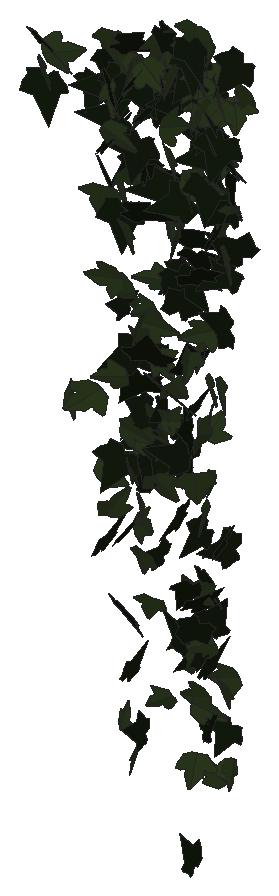
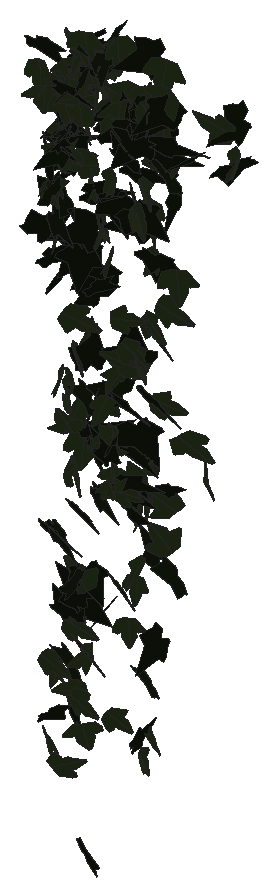
# SketchUp Ruby script. Lengths in millimetres.
U = 1.mm
M = Sketchup.active_model
def pt(a) = Geom::Point3d.new(a.map { |v| v * U })
def face(e, loops, mat)
  f = e.add_face(loops[0].map { |a| pt(a) })
  loops[1..].each { |l| e.add_face(l.map { |a| pt(a) }).erase! }
  f.material = f.back_material = mat if mat
  f
end
# faces: each face lists its corners as indices into pts; further lists are holes
def faces(e, pts, list, mat = nil) = list.each { |f| face(e, (f[0].is_a?(Array) ? f : [f]).map { |l| l.map { |i| pts[i] } }, mat) }
# xy, xz, yz: faces in a plane at the given z, y or x. An outline is a flat list of corners, or four numbers for a rectangle; further outlines are holes
def ring(l) = l.size == 4 ? [[l[0], l[1]], [l[2], l[1]], [l[2], l[3]], [l[0], l[3]]] : l.each_slice(2).to_a
def flat(e, list, mat, &to3) = list.each { |f| face(e, (f[0].is_a?(Array) ? f : [f]).map { |l| ring(l).map { |u, v| to3.(u, v) } }, mat) }
def xy(e, z, list, mat = nil) = flat(e, list, mat) { |x, y| [x, y, z] }
def xz(e, y, list, mat = nil) = flat(e, list, mat) { |x, z| [x, y, z] }
def yz(e, x, list, mat = nil) = flat(e, list, mat) { |y, z| [x, y, z] }
def lines(e, pts, list) = list.each { |a, b| e.add_line(pt(pts[a]), pt(pts[b])) }
# prism: a flat outline (further loops are holes) pulled along v
def prism(e, loops, v, mat = nil)
  f = face(e, loops, mat); d = Geom::Vector3d.new(v.map { |x| x * U })
  f.pushpull(f.normal.samedirection?(d) ? d.length : -d.length)
end
def box(e, o, s, mat = nil) = prism(e, [[o, [o[0] + s[0], o[1], o[2]], [o[0] + s[0], o[1] + s[1], o[2]], [o[0], o[1] + s[1], o[2]]]], [0, 0, s[2]], mat)
def at(x, y, z, deg = 0) = Geom::Transformation.translation(pt([x, y, z])) * Geom::Transformation.rotation(ORIGIN, Z_AXIS, deg.degrees)
def axes(o, x, y, z) = Geom::Transformation.new([*x, 0, *y, 0, *z, 0, *pt(o).to_a, 1])
def part(name) = M.definitions.add(name)
# library, detail: a bought-in or finely detailed component or shape, given as its bounding box
def library(name, o, s) = part(name).tap { |d| box(d.entities, o, s) }
def detail(e, o, s) = box(e.add_group.entities, o, s)
def put(e, d, t, mat = nil) = e.add_instance(d, t).tap { |i| i.material = mat if mat }
def group(e, t, mat = nil) = e.add_group.tap { |g| g.transformation = t; g.material = mat if mat }.entities
root = M.entities
M.materials.add("efeu1").color = [18, 25, 13]
M.materials.add("efeu2").color = [43, 57, 29]
c1 = part("ivyleaf_9")
p = [[39.1,54.8,31.7],[34.5,51.8,30.2],[-5.3,25.2,17.3],[-17.9,28.3,20.9],[-21.6,21.7,17],[-20.2,4.3,5.3],
  [-22.9,-0.3,2.5],[-17.1,-4,-0.6],[-2,-2.1,-1.2],[-0.7,-15.4,-10.1],[16.6,-22.3,-16.7],[21.1,-15.1,-12.5],
  [32.7,-10.7,-11],[46.1,-1.8,-6.6],[30.8,11.2,3.8]]
faces(c1.entities,p,[[0,1,2,3,4,5,6,7,8,9,10,11,12,13,14]],"efeu1")
c2 = part("ivyleaf_10")
p = [[0,12.8,-0.8],[-1.5,51.3,-10.9],[-4.9,51,-11.6],[-13.6,26.5,-7.3],[-13.2,15.9,-4.6],[-21.1,19.3,-7.2],
  [-29.5,16.3,-8.3],[-29.2,8.3,-6.2],[-19.7,-9.8,0.5],[-7.6,-13,4],[1,-12.2,5.8],[-0.4,51.1,-11.1],
  [-1.5,51.1,-10.9],[1,-12.4,5.9],[16.9,-12.4,3.5],[35.1,9.1,-5.1],[35,12.9,-6.1],[20.5,16.4,-4.9],
  [15.8,15,-3.8],[15.3,27.6,-7.1],[12.8,31.3,-7.8]]
faces(c2.entities,p,[[0,1,2,3,4,5,6,7,8,9,10],[11,12,0,13,14,15,16,17,18,19,20]],"efeu2")
put(root,c1,axes([688.2,842.5,1500.4],[-0.57165,0.78495,-0.04748],[0.02556,-0.04278,-0.91416],[-0.95905,-0.46901,0.00394]))
put(root,c2,axes([645.1,855.7,237.5],[0.35837,-0.69674,0.27974],[0.154,-0.25029,-0.75591],[0.90294,0.31922,0.0179]))
put(root,c1,axes([575,857.3,1511.8],[-0.02419,0.00992,-0.97393],[1.18118,-0.10596,-0.02079],[-0.12949,-0.96835,-0.0077]))
put(root,c2,axes([723.9,861.1,1577.1],[0.29067,-0.90245,0.42845],[0.13727,-0.41342,-0.93336],[1.21101,0.26347,0.00296]))
put(root,c1,axes([663.5,857.4,1001],[1.24622,0.12938,0.36273],[-0.44106,-0.03213,1.02957],[0.16188,-1.0835,0.01278]))
put(root,c2,axes([591.8,850.9,1419.5],[-0.56354,0.07919,-0.839],[1.00063,-0.17754,-0.46832],[-0.23618,-0.94115,0.01775]))
put(root,c1,axes([445.5,860.4,1465],[-0.21538,-1.02923,-0.21362],[0.04513,0.21039,-1.04426],[1.28163,-0.18037,0.00088]))
put(root,c1,axes([581.1,841.8,1349.9],[0.75889,-0.1453,-0.68342],[-0.78059,0.24916,-0.63534],[0.34246,0.8899,0.0663]))
put(root,c1,axes([435.1,846.9,1550.6],[1.27473,-0.33971,-0.04287],[-0.05146,0.00891,-1.09869],[0.41455,1.04571,-0.00457]))
put(root,c1,axes([746.5,865.5,833.4],[-0.26063,-0.06395,0.97431],[-1.07992,-0.40825,-0.22088],[0.50276,-0.91008,0.03062]))
put(root,c2,axes([775.6,851,811.5],[-0.87861,-0.76846,-0.08968],[0.10941,0.03878,-1.05246],[0.93752,-0.7247,0.03878]))
put(root,c2,axes([729.6,832.1,1480.4],[-0.0609,0.28687,1.01127],[-0.19448,0.99864,-0.29116],[-1.2676,-0.167,-0.00391]))
put(root,c2,axes([605,860.6,945.7],[-0.1939,-0.07915,0.84036],[-0.83265,-0.4911,-0.17534],[0.60592,-0.70021,0.02798]))
put(root,c2,axes([794.5,855.9,752.1],[0.59858,-0.8846,-0.06879],[-0.02613,0.06677,-1.01146],[1.08215,0.49092,0.01363]))
put(root,c1,axes([648.7,870.1,266.9],[-0.13054,-0.05321,0.83212],[-0.45682,-0.74653,-0.09589],[0.90892,-0.38285,0.07132]))
put(root,c1,axes([637.4,859.6,1529.6],[-0.5503,0.60726,-0.57818],[0.38588,-0.48479,-0.75594],[-0.94738,-0.5502,0.02794]))
put(root,c1,axes([624.3,840.8,1605],[0.84106,0.31815,0.61576],[0.69981,0.22558,-0.75877],[-0.47462,0.8964,-0.0276]))
put(root,c2,axes([546.6,861.3,892.8],[0.9218,0.18129,-0.74961],[-0.8839,-0.19283,-0.77691],[-0.32249,1.04672,-0.01329]))
put(root,c1,axes([612.9,853,638.5],[0.22219,0.79996,0.34057],[-0.09776,-0.33103,0.82042],[1.0562,-0.19892,0.00429]))
put(root,c2,axes([596.9,854.6,1601.3],[-1.27596,-0.14242,-0.04362],[0.06573,-0.07332,-1.05249],[0.16941,-1.04421,0.07985]))
put(root,c2,axes([595.1,855.4,1133.6],[0.35201,0.0285,-0.97971],[-1.16682,0.23149,-0.27493],[0.26145,0.99473,0.09206]))
put(root,c2,axes([622.8,871.8,1537.8],[-0.06106,0.49555,-0.81179],[0.01845,-0.81239,-0.49685],[-1.16018,-0.039,0.03482]))
put(root,c1,axes([638.5,847.7,1282.1],[0.90202,0.13135,0.63669],[0.76026,0.13147,-0.75078],[-0.22593,0.96682,0.0156]))
put(root,c1,axes([743.8,877.4,877.8],[-0.14166,-0.09459,0.97914],[-0.21184,-0.96848,-0.11415],[1.18126,-0.18502,0.09695]))
put(root,c2,axes([462.3,857.3,1524.4],[0.47885,-0.06622,-1.01584],[1.23901,-0.04945,0.39562],[-0.08546,-1.0879,0.04385]))
put(root,c2,axes([723.8,869.9,1262.1],[0.54561,-0.80603,0.40219],[0.23354,-0.35374,-0.92178],[1.07387,0.48645,-0.00388]))
put(root,c1,axes([739.8,862.9,726.6],[-0.81189,0.50808,-0.34511],[0.30124,-0.2446,-0.83625],[-0.6861,-0.70862,0.04122]))
put(root,c1,axes([582.5,846.8,1387.1],[-0.3417,0.92287,-0.00056],[-0.00222,0.00003,0.96443],[1.1259,0.28008,0.00173]))
put(root,c2,axes([643.1,865.7,718.4],[-0.37225,0.63443,-0.4362],[0.22794,-0.39416,-0.70399],[-0.91122,-0.35778,0.0021]))
put(root,c1,axes([633.1,849.7,383.9],[-0.52443,0.75206,0.02487],[-0.00429,-0.03065,0.86605],[0.918,0.42949,0.01825]))
put(root,c1,axes([599.7,875.6,783.9],[-0.80764,-0.7157,0.0618],[-0.05389,-0.04332,-0.97491],[0.87474,-0.66347,-0.003]))
put(root,c1,axes([824.7,877.5,1105.9],[0.12813,-0.94989,-0.2167],[0.18779,-0.19904,0.94709],[-1.17372,-0.13554,0.12788]))
put(root,c2,axes([764.3,865.1,257.5],[0.80321,0.68502,-0.18949],[-0.15952,-0.13715,-0.95011],[-0.85231,0.67123,-0.00075]))
put(root,c1,axes([598.3,872,1437.2],[-0.42262,-0.35025,-0.80445],[-0.65794,-0.59722,0.49225],[-0.84434,0.64068,0.01908]))
put(root,c1,axes([817.4,873.5,1467],[-0.98561,-0.56282,-0.29022],[0.30299,0.15116,-0.98445],[0.71066,-0.84501,0.0172]))
put(root,c2,axes([589.9,866.1,1494.6],[0.49854,0.86846,-0.1499],[-0.07238,-0.13775,-0.95978],[-1.07275,0.41289,-0.00491]))
put(root,c2,axes([609.4,864,274.9],[0.81494,-0.44559,-0.00085],[0.00804,0.00835,0.8029],[-0.54356,-0.66793,0.0106]))
put(root,c1,axes([736.9,869.5,474.2],[-0.07849,-0.83718,0.30362],[0.02641,0.30285,0.83965],[-1.08614,0.06786,-0.00153]))
put(root,c2,axes([748.2,873.3,1033.2],[0.00036,0.88393,-0.54042],[-0.12167,-0.53789,-0.87984],[-1.25811,0.05227,0.08493]))
put(root,c2,axes([433.9,864.9,1483.2],[-0.75237,0.84837,-0.22552],[0.184,-0.16911,-1.0486],[-1.05503,-0.63449,-0.02206]))
put(root,c2,axes([581.3,855.7,746.6],[0.68104,0.35764,-0.70091],[0.73054,0.36446,0.66287],[0.62281,-0.81857,-0.0111]))
put(root,c1,axes([738.1,882.3,1319.1],[-0.6916,-0.33915,0.724],[-0.76747,-0.35855,-0.66051],[0.60198,-0.84675,-0.0103]))
put(root,c2,axes([608.4,866.7,1231.4],[-0.81188,0.50109,-0.25611],[0.25536,-0.14777,-0.83301],[-0.63729,-0.69758,-0.00751]))
put(root,c1,axes([577.6,849,612.9],[-0.60714,0.87211,-0.31711],[-0.19182,0.27538,1.00411],[1.11576,0.5219,0.00007]))
put(root,c2,axes([687.1,862.8,773.3],[-0.98838,-0.24989,-0.44222],[0.50581,0.15561,-0.84748],[0.358,-0.90977,-0.02349]))
put(root,c1,axes([690.9,867,1638],[0.79503,-0.72239,-0.34968],[-0.2002,0.321,-0.96893],[0.95845,0.66626,0.08768]))
put(root,c1,axes([779.1,880.5,1369.7],[-0.32014,-0.95865,-0.10441],[0.02087,0.10356,-0.99385],[1.17628,-0.26275,-0.01079]))
put(root,c2,axes([583,865,676.3],[-0.40517,-0.84542,0.42958],[0.18791,0.40103,0.9083],[-1.14156,0.36607,-0.00296]))
put(root,c1,axes([758.6,879.2,510.5],[0.07301,0.23906,-0.85319],[-0.17985,-0.84053,-0.24586],[-1.06591,0.15819,-0.01696]))
put(root,c1,axes([765,854.9,1198],[0.89903,0.68881,0.20241],[0.17951,0.139,-1.0087],[-0.85728,0.75145,0.00104]))
put(root,c2,axes([683.8,871.1,1622.4],[-0.36371,-0.9845,-0.10293],[0.05545,0.09377,-1.02852],[1.20637,-0.30113,0.01625]))
put(root,c1,axes([631.2,880.4,1399.1],[-0.89009,-0.54805,-0.39857],[0.43458,0.18806,-0.91063],[0.70331,-0.8098,0.05826]))
put(root,c1,axes([675.1,877.5,947],[0.74478,-0.69246,0.52491],[0.63676,-0.22066,-0.89812],[0.84754,0.77429,0.21349]))
put(root,c1,axes([618.8,866.4,1087.3],[-0.63764,0.60055,0.31657],[-0.25764,0.23588,-0.79612],[-0.78714,-0.56369,0.00413]))
put(root,c1,axes([747.4,890.2,1571.3],[-0.73683,-0.68215,0.21429],[-0.07461,-0.2302,-0.90515],[0.86913,-0.59808,0.10397]))
put(root,c1,axes([745.7,861.3,800],[-0.09104,0.19995,0.88238],[-0.40022,0.81915,-0.21337],[-1.02868,-0.3364,0.00492]))
put(root,c1,axes([743,884.7,1602.2],[-0.23918,-0.91452,-0.13606],[0.03625,0.13278,-0.9353],[1.12741,-0.19829,0.00121]))
put(root,c2,axes([757.5,879.8,1556.7],[1.04657,0.50845,-0.2865],[-0.31655,-0.12396,-0.9969],[-0.63776,0.89588,0.02466]))
put(root,c2,axes([618.2,873.3,1106.8],[-0.49484,0.08531,0.80091],[-0.97766,0.04734,-0.41088],[-0.09871,-0.89651,0.05451]))
put(root,c1,axes([738,884.2,1621.6],[0.13618,-0.92575,-0.17275],[0.05295,0.17883,-0.93029],[1.14769,0.10159,0.06342]))
put(root,c1,axes([770.1,883,696.5],[-1.03787,0.12254,-0.19994],[0.23764,-0.0497,-0.85924],[-0.15931,-0.87248,0.02086]))
put(root,c2,axes([604.7,877.8,835.6],[0.02578,-0.07274,0.90666],[1.09988,0.12189,-0.01123],[-0.14709,0.89867,0.07491]))
put(root,c2,axes([619.6,870.5,766.7],[-0.71731,0.45142,0.38745],[-0.3805,0.22997,-0.74123],[-0.61802,-0.66552,0.00666]))
put(root,c2,axes([611.9,862.9,1287.3],[-0.1889,0.42908,-0.88912],[-0.47485,0.80056,0.45412],[1.10688,0.41667,0.04308]))
put(root,c1,axes([721.3,875.1,1177.7],[-0.29148,-0.3734,-0.91187],[0.59987,0.76795,-0.44329],[1.04178,-0.54667,0.00013]))
put(root,c1,axes([731,866.4,1115.9],[-0.34567,-0.18318,0.99106],[1.04117,0.50402,0.33715],[-0.65406,0.89913,0.01291]))
put(root,c2,axes([747.8,870.3,1365.5],[0.15328,0.11221,0.99196],[0.96683,0.59677,-0.16788],[-0.74063,0.80226,-0.01386]))
put(root,c1,axes([620.7,877.3,1517.1],[-0.02422,-0.73608,-0.71535],[0.08628,0.7128,-0.73542],[1.24926,-0.0635,0.03692]))
put(root,c1,axes([730.1,888.3,995.2],[0.63864,0.52675,0.70252],[-0.57822,-0.51901,0.74231],[0.90179,-0.70583,-0.02155]))
put(root,c1,axes([744.2,881.3,580.8],[0.23757,0.6141,-0.59155],[-0.20444,-0.56738,-0.64418],[-1.01997,0.25676,-0.00866]))
put(root,c1,axes([592.2,873.6,493.6],[1.16212,-0.13069,-0.37223],[-0.44275,0.0912,-0.96072],[0.18874,1.01863,0.03826]))
put(root,c2,axes([715.2,877.1,1605.6],[0.31169,0.99358,0.11453],[0.05415,0.10683,-1.02577],[-1.21899,0.2588,-0.01628]))
put(root,c1,axes([588.1,895.4,1505.3],[-0.30607,-0.99837,0.03488],[-0.01425,-0.03302,-1.0294],[1.21867,-0.25113,-0.00328]))
put(root,c2,axes([811.8,883.4,1243.5],[-0.49094,0.84864,-0.31541],[0.20166,-0.27049,-0.93867],[-1.08597,-0.43388,-0.03172]))
put(root,c2,axes([763.6,898.3,1538.4],[-0.23231,-0.68735,0.71283],[0.20335,-0.73778,-0.66688],[1.19086,-0.0081,0.25294]))
put(root,c2,axes([731.3,887.2,1579.1],[-0.81305,-0.64585,0.35343],[-0.28316,-0.2681,-0.92759],[0.85239,-0.7051,0.02897]))
put(root,c1,axes([804.3,862.4,1279.6],[0.03497,0.57602,0.83709],[-0.04228,0.83749,-0.57511],[-1.23895,-0.01232,0.04325]))
put(root,c2,axes([632.7,886.3,1009],[-0.93403,0.14191,0.40034],[0.4797,-0.07534,0.77863],[0.196,0.86066,0.00215]))
put(root,c2,axes([800.5,887.3,1523.5],[1.02428,0.22222,-0.52805],[-0.64314,-0.06716,-0.86642],[-0.27367,0.98955,0.05978]))
put(root,c1,axes([699.9,889.7,1560],[0.54745,-0.83246,-0.02957],[-0.00737,0.03033,-0.94565],[1.01621,0.44868,0.00907]))
put(root,c2,axes([467.3,896.7,852.7],[0.45747,-0.24571,0.89672],[0.90798,-0.50024,-0.44829],[0.67991,0.83336,-0.00469]))
put(root,c2,axes([745.9,870.7,1334.7],[-0.08743,0.0519,1.0062],[-1.01545,0.56538,-0.08845],[-0.69266,-0.83541,0.00266]))
put(root,c1,axes([587.6,890.7,1250.8],[-0.87534,-0.43155,-0.60235],[0.62878,0.31176,-0.83727],[0.6495,-0.88341,-0.00123]))
put(root,c2,axes([608.8,876.9,1335.2],[-0.46065,-0.60266,-0.50523],[0.35835,0.41181,-0.71075],[0.89,-0.47774,0.02468]))
put(root,c1,axes([750.2,896.3,1565.3],[-0.8785,-0.57871,-0.0922],[0.07681,0.06882,-0.9237],[0.7108,-0.72269,-0.01414]))
put(root,c1,axes([779.6,901.4,1412.9],[-0.68107,-0.20289,0.73166],[-0.7015,-0.4801,-0.57186],[0.60494,-0.78516,0.16061]))
put(root,c2,axes([650.3,876.4,1548.8],[0.58828,0.75936,0.55764],[0.36647,0.46983,-0.89952],[-1.0894,0.5681,-0.00147]))
put(root,c2,axes([769.4,893.1,470.6],[-0.4258,-0.10855,0.79418],[-0.80023,-0.45919,-0.35103],[0.56208,-0.73599,0.10187]))
put(root,c1,axes([696.3,904,1486.8],[-0.2214,-0.23236,0.82745],[-0.69511,-0.60063,-0.29362],[0.78502,-0.59737,-0.02662]))
put(root,c1,axes([681.6,899.2,1317.1],[-0.66432,-0.15865,0.72889],[-0.85176,-0.20942,-0.56716],[0.3205,-0.8854,0.00354]))
put(root,c2,axes([604.6,899.1,1539.7],[-0.34626,-0.69428,0.42901],[0.22697,-0.45744,-0.68972],[1.53661,-0.08888,0.19855]))
put(root,c1,axes([522.2,905,1461.2],[-0.42809,-0.6929,0.37191],[-0.24891,-0.34848,-0.72834],[1.47584,-0.25976,-0.01496]))
put(root,c2,axes([770,894.7,1074],[0.50247,0.20026,-0.86069],[-1.03885,-0.16391,-0.44561],[-0.28821,0.93997,0.10566]))
put(root,c1,axes([743.5,875.3,913.3],[-0.42711,0.82077,-0.14824],[-0.07317,0.13558,0.89231],[1.0149,0.35518,0.00195]))
put(root,c2,axes([633.7,887,598.3],[-0.93962,0.15489,0.15891],[-0.19396,0.01531,-0.78544],[-0.18888,-0.78626,0.01601]))
put(root,c1,axes([786.7,892.5,1452.5],[0.75203,-0.76466,-0.13822],[-0.11664,0.10045,-0.98211],[0.9408,0.62368,-0.01128]))
put(root,c1,axes([727.9,880.1,1248.2],[0.98482,0.10253,0.55951],[0.67448,0.08718,-0.8136],[-0.16332,0.9783,0.01387]))
put(root,c2,axes([767.7,873.7,884],[-0.04642,-0.46494,-0.9417],[0.11173,0.93726,-0.46644],[1.27639,-0.09895,0.00658]))
put(root,c1,axes([573.6,899,1476.9],[-0.89743,0.05233,0.71313],[-0.87211,-0.078,-0.73164],[0.02062,-1.02155,0.0924]))
put(root,c1,axes([803.6,911.4,1321.3],[-0.40073,-0.57411,0.70321],[-0.25161,-0.68108,-0.65238],[1.07856,-0.37219,0.10909]))
put(root,c1,axes([609.9,893.4,978.6],[-1.1691,0.35686,0.14479],[-0.15834,0.06631,-1.02244],[-0.44236,-0.96689,-0.01668]))
put(root,c2,axes([566.3,889.4,1569.4],[-0.97334,0.07041,-0.65551],[0.79616,-0.06194,-0.80091],[-0.11434,-1.03071,0.00335]))
put(root,c2,axes([648.4,891.8,513],[-0.89435,-0.23476,0.16603],[-0.19188,-0.05326,-0.76974],[0.29367,-0.74975,0.00269]))
put(root,c2,axes([620.8,898.7,1046.5],[0.48898,-0.92985,0.14758],[0.07203,-0.13526,-1.01255],[1.14636,0.40513,0.00068]))
put(root,c2,axes([740.5,894.5,560.9],[-0.83806,-0.1987,0.67991],[0.83323,0.06545,0.70916],[-0.22924,0.9643,0.09196]))
put(root,c2,axes([673,883.2,992.3],[0.20006,0.79246,0.40546],[0.05143,0.40491,-0.80842],[-1.08478,0.16535,0.03645]))
put(root,c2,axes([803.1,881.7,1537.9],[-0.6423,0.64251,0.59147],[-0.53997,0.39906,-0.82746],[-0.91847,-0.68393,0.07284]))
put(root,c1,axes([736.7,903.6,1565.9],[-1.07247,-0.24823,0.16724],[-0.20294,-0.02618,-0.91323],[0.30357,-0.89445,-0.01968]))
put(root,c2,axes([808,902.4,1315.6],[-0.21775,-0.85958,0.319],[0.013,-0.32691,-0.87494],[1.1185,-0.16355,0.07227]))
put(root,c2,axes([778.2,882,1499.5],[-0.28,-0.39398,0.86214],[0.45644,0.77738,0.45484],[-1.06254,0.43776,-0.0318]))
put(root,c1,axes([765.1,902.1,1464.6],[-1.03616,0.02372,-0.32348],[0.39245,-0.05452,-0.84858],[-0.05068,-0.90719,0.04254]))
put(root,c1,axes([667.7,911.8,794.9],[-0.4612,-0.81439,0.26484],[0.03976,-0.30297,-0.88512],[1.04402,-0.34823,0.15071]))
put(root,c1,axes([707,910.8,1159.3],[-0.49667,-0.56027,0.44435],[-0.33376,-0.35039,-0.69244],[0.80604,-0.49032,-0.01292]))
put(root,c1,axes([754.8,900.5,297.9],[-0.14752,0.37533,0.76142],[0.28505,-0.72469,0.39433],[0.99566,0.26308,-0.00008]))
put(root,c2,axes([752.5,889.3,345.5],[0.23458,0.07049,0.84959],[0.90777,0.41121,-0.20252],[-0.50763,0.76791,0.03045]))
put(root,c1,axes([720.8,879.5,1607.2],[0.06196,1.00163,0.2455],[-0.18246,0.25035,-0.99049],[-1.24486,0.01316,0.1574]))
put(root,c1,axes([741.4,891.2,533.7],[0.692,0.75796,0.02512],[-0.02245,-0.0176,0.94669],[0.92495,-0.5675,0.00419]))
put(root,c2,axes([753,891.9,1571],[-0.50325,0.83818,0.00581],[-0.0081,0.00321,-0.93417],[-1.02257,-0.41253,0.00454]))
put(root,c1,axes([758.8,906.8,1526],[0.20097,-0.99684,0.05025],[0.01128,-0.04941,-1.01036],[1.21764,0.16498,0.00107]))
put(root,c1,axes([764.2,905.9,1445.2],[0.03279,-0.00182,0.92759],[0.55453,-0.80891,-0.01476],[0.98649,0.45477,-0.02253]))
put(root,c2,axes([744.6,894.5,1483.3],[0.6838,-0.62433,-0.35969],[-0.26932,0.28498,-0.83867],[0.83677,0.60192,0.02399]))
put(root,c2,axes([725.7,898.4,1570.7],[1.07761,0.30052,-0.02109],[-0.02242,-0.01147,-0.933],[-0.36685,0.88347,-0.00494]))
put(root,c2,axes([764.8,897.5,1573.7],[0.49275,0.90655,-0.10831],[-0.01872,-0.11168,-0.99196],[-1.1137,0.40297,-0.03125]))
put(root,c2,axes([770.9,897.1,1616.8],[0.66557,-0.768,-0.16209],[-0.08613,0.15743,-0.84355],[1.49138,0.35183,0.02362]))
put(root,c1,axes([766.9,913.1,1454.8],[0.04772,-0.90435,0.36839],[0.128,-0.36266,-0.90142],[1.18443,0.07562,0.08257]))
put(root,c1,axes([640.9,885.2,1350.3],[-0.21259,0.0591,-0.95216],[-1.09519,0.31742,0.18399],[0.39389,0.91445,-0.00233]))
put(root,c1,axes([648.9,898.1,775.5],[-0.45595,-0.15928,-0.74864],[-0.85804,-0.25723,0.40582],[-0.36841,0.79622,-0.01865]))
put(root,c2,axes([653.4,900.8,859.4],[-0.78699,-0.01848,0.55003],[0.67105,0.00643,0.6453],[-0.02224,0.84771,0.0071]))
put(root,c2,axes([671.8,904.4,329.5],[-0.44101,-0.24223,0.61925],[-0.61514,-0.35964,-0.43502],[0.52886,-0.62032,0.0104]))
put(root,c2,axes([761.3,913.8,773.9],[0.04755,-0.06049,0.83472],[0.51351,-0.72083,-0.07189],[0.8825,0.4227,-0.00314]))
put(root,c1,axes([752.5,900.9,449.2],[-1.02983,0.47718,-0.05622],[0.05873,-0.02908,-0.96966],[-0.58323,-0.84549,0.00162]))
put(root,c2,axes([753.9,905.9,1443.5],[-0.50625,0.4921,-0.58637],[0.48757,-0.4296,-0.64335],[-0.79653,-0.57573,-0.02113]))
put(root,c2,axes([773.5,901.2,1496.7],[-1.02524,-0.47868,0.15039],[-0.16018,-0.07334,-0.96713],[0.5908,-0.85056,-0.00124]))
put(root,c2,axes([689.4,912.7,1571.3],[0.49852,-0.76731,0.42353],[0.25696,-0.36764,-0.86926],[1.03792,0.45956,0.01177]))
put(root,c1,axes([562.6,886,1551.5],[0.02479,-0.08776,-1.04254],[-0.07462,1.04085,-0.08881],[1.27421,0.06266,0.01508]))
put(root,c2,axes([599.6,887.1,1512.6],[-0.07017,0.57676,-0.73354],[-0.10658,0.72837,0.57955],[1.13342,0.1042,0.00909]))
put(root,c2,axes([806.9,909,243.6],[0.8052,-0.412,0.30493],[0.30628,-0.17358,-0.77792],[0.54518,0.70601,-0.01332]))
put(root,c2,axes([759.1,914.8,906.8],[0.19601,-0.52835,-0.63071],[0.22697,-0.60265,0.55223],[-0.97778,-0.2458,0.00175]))
put(root,c1,axes([658.1,919.7,874.4],[0.30073,-0.47253,-0.63524],[0.464,-0.51285,0.52907],[-0.84715,-0.44864,0.06428]))
put(root,c1,axes([799.7,920.1,1189.8],[-0.65075,-0.52045,0.56705],[-0.50411,-0.38843,-0.74519],[0.79223,-0.67468,-0.0084]))
put(root,c2,axes([726.9,892.7,1597],[0.43273,0.64192,0.56881],[0.31165,0.50853,-0.73318],[-0.99887,0.43675,0.01767]))
put(root,c1,axes([628.9,911.4,868.2],[-1.16661,-0.08571,-0.10025],[0.12372,-0.00865,-0.95991],[0.10288,-0.96144,0.01757]))
put(root,c1,axes([640.6,896.9,737.8],[-0.30644,0.27057,0.71602],[-0.59385,0.52511,-0.36919],[-0.72068,-0.54775,-0.00024]))
put(root,c2,axes([773.3,906.8,1439.7],[1.10562,0.11586,-0.09509],[-0.1167,-0.00159,-0.91356],[-0.14079,0.91122,0.0105]))
put(root,c1,axes([765,908.9,1454.2],[0.73093,-0.673,0.08127],[0.06943,-0.05814,-0.90104],[0.82411,0.60181,0.00383]))
put(root,c1,axes([612.8,914,1340.3],[0.0782,0.31215,-0.93065],[-0.30062,-0.89765,-0.31806],[-1.15922,0.25385,0.0197]))
put(root,c1,axes([798.9,914.2,1346.5],[-0.21714,0.33647,0.88831],[0.18008,-0.88299,0.36404],[1.1448,0.20272,0.11123]))
put(root,c1,axes([656.8,896.3,1534.2],[0.18603,0.05484,-0.92547],[-1.12756,0.08265,-0.14738],[0.08882,0.9343,0.06736]))
put(root,c1,axes([823.1,915.2,1600.6],[-1.13499,-0.26697,-0.1007],[0.11472,0.03737,-0.96782],[0.32865,-0.93501,-0.00993]))
put(root,c1,axes([742.3,898.3,1212],[0.8323,0.51339,-0.45747],[-0.46713,-0.25165,-0.85342],[-0.69683,0.7819,0.0257]))
put(root,c1,axes([821,916.5,1229.3],[0.19686,0.04894,0.94365],[-1.12513,-0.20032,0.16809],[0.25104,-0.93616,0.01336]))
put(root,c2,axes([637.7,907.9,1062.2],[-0.5089,-0.07572,0.75812],[-0.90369,-0.16199,-0.42374],[0.21755,-0.85,0.01322]))
put(root,c2,axes([737.4,905.3,1566.1],[-1.0406,0.31445,0.19322],[-0.28137,-0.07428,-0.89723],[-0.35152,-0.8714,0.1462]))
put(root,c1,axes([764.4,904.5,495.9],[-0.67014,0.21702,0.62365],[0.65093,-0.33209,0.5855],[0.47464,0.76183,0.07757]))
put(root,c2,axes([670.8,906.9,1381.5],[-0.7694,0.60577,-0.2107],[0.1733,-0.15624,-0.87435],[-0.76304,-0.6463,0.01388]))
put(root,c2,axes([643.7,913.2,779.8],[-0.06953,0.04209,0.78568],[-0.82549,-0.40464,-0.02741],[0.48988,-0.67588,0.06534]))
put(root,c1,axes([749,922.1,1436.6],[-0.64259,-0.71516,0.08034],[0.03309,-0.11922,-0.88339],[0.87736,-0.5193,0.09216]))
put(root,c2,axes([709.6,896.1,1538.4],[-0.42432,0.50117,0.6409],[-0.54024,0.46811,-0.60636],[-0.83267,-0.5591,0.06681]))
put(root,c2,axes([667.1,909.5,791.5],[0.31651,0.7715,-0.15752],[-0.07478,-0.14556,-0.81387],[-0.95773,0.26633,0.01149]))
put(root,c1,axes([772.1,904,1454.3],[0.90107,-0.38363,-0.39965],[-0.44083,0.17126,-0.83217],[0.5123,0.82213,-0.01314]))
put(root,c2,axes([752.5,917.4,958.7],[-0.28824,0.36051,-0.71898],[0.50404,-0.58854,-0.43087],[-0.84189,-0.47579,-0.0118]))
put(root,c2,axes([728.6,909.9,1635.4],[-1.125,-0.11223,0.20381],[-0.22462,-0.15731,-0.91968],[0.17354,-0.93119,0.1308]))
put(root,c1,axes([663.1,904.7,1342.9],[0.43111,0.53975,-0.61882],[-0.69073,-0.32779,-0.60921],[-0.72558,0.63274,0.21227]))
put(root,c1,axes([734,896.8,32.6],[-0.14349,0.29479,0.87947],[-0.44597,0.80004,-0.31705],[-1.04005,-0.38373,0.01461]))
put(root,c2,axes([628,907.8,1032.4],[-0.13525,-0.02441,1.00018],[1.16922,0.28626,0.11321],[-0.35035,0.96473,-0.00829]))
put(root,c1,axes([723.5,926.8,1554],[-0.0848,-0.29116,0.81802],[0.10375,-0.81898,-0.28428],[1.05423,0.05717,0.09377]))
put(root,c2,axes([614.6,902,810],[0.16723,0.03484,0.93038],[0.88349,0.58705,-0.12867],[-0.71388,0.73469,0.0587]))
put(root,c2,axes([645.7,920.7,1121.2],[0.04539,0.01773,0.81143],[-0.68618,-0.58506,0.03858],[0.71388,-0.56348,-0.01452]))
put(root,c1,axes([791.4,925,305],[-0.43673,-0.69155,0.18575],[-0.10715,-0.1637,-0.7787],[0.867,-0.36858,-0.00267]))
put(root,c2,axes([780.1,924.1,1238.1],[-0.19705,0.36295,-0.78469],[0.33568,-0.73518,-0.39669],[-0.99992,-0.31833,0.02147]))
put(root,c2,axes([685.2,904.5,937.1],[-0.45569,-0.60882,-0.48516],[0.3104,0.4131,-0.71427],[0.8976,-0.45194,0.0007]))
put(root,c2,axes([787.1,909.3,390.8],[-0.84848,0.46011,-0.04222],[0.03981,-0.0272,-0.83389],[-0.56229,-0.69622,0.00467]))
put(root,c2,axes([681.4,897.2,869.2],[0.13749,0.18418,0.78639],[0.16412,0.77864,-0.20165],[-0.9716,0.15759,0.07722]))
put(root,c2,axes([692.2,916.8,1255.7],[-0.54065,0.71475,0.31559],[0.19409,-0.27267,0.84094],[0.93324,0.47078,0.00793]))
put(root,c1,axes([750.7,916.9,1435.3],[0.06638,-0.92264,-0.35375],[-0.04694,0.35204,-0.9241],[1.20461,0.06456,-0.01652]))
put(root,c2,axes([739.9,917.8,1023.8],[0.72426,-0.73168,0.1017],[0.07826,-0.07892,-0.94223],[0.89783,0.59711,0.00009]))
put(root,c2,axes([768.9,913.6,1405.3],[1.13967,0.2815,0.13783],[0.15586,0.05369,-0.97554],[-0.34918,0.94274,0.01441]))
put(root,c1,axes([632.2,924.6,809.6],[-0.86824,-0.22359,0.5145],[-0.59632,-0.16072,-0.74595],[0.33588,-0.86334,0.00562]))
put(root,c1,axes([607.5,915.1,921.3],[0.30948,0.55947,-0.77825],[-0.38602,-0.71103,-0.61429],[-1.10379,0.40553,-0.00338]))
put(root,c2,axes([727,915.9,1483.9],[-1.10999,-0.09972,0.23756],[0.28795,0.02702,0.91528],[-0.12604,0.93994,-0.00111]))
put(root,c2,axes([730.2,896.8,428],[-0.0298,-0.07854,-0.94323],[0.3201,0.906,-0.08224],[1.10947,-0.26351,-0.0016]))
put(root,c2,axes([776.7,914.8,961.8],[-0.42462,0.85303,-0.18752],[0.08749,-0.17326,-0.9213],[-1.06194,-0.35536,-0.00093]))
put(root,c2,axes([774.9,919.8,203.5],[0.41583,0.34409,0.74858],[-0.77166,-0.40983,0.47637],[0.64408,-0.71316,0.08743]))
put(root,c1,axes([646.8,927.4,1505.8],[-0.93579,-0.5943,-0.02832],[0.02515,0.01963,-0.97033],[0.72543,-0.76731,-0.00289]))
put(root,c1,axes([659.4,907.7,596.4],[-0.51984,0.54584,0.35352],[-0.24606,0.29088,-0.69223],[-0.75427,-0.47108,-0.01782]))
put(root,c1,axes([668,918.2,840.8],[-0.29815,0.1777,0.76249],[0.65211,-0.54578,0.29851],[0.69792,0.58587,0.04682]))
put(root,c1,axes([805.9,915.4,656.8],[-0.93299,0.40091,0.35041],[-0.40696,0.11726,-0.86216],[-0.50633,-0.83299,0.04728]))
put(root,c1,axes([784.5,929.6,1320.4],[0.23411,-0.53853,0.65934],[0.39868,-0.57751,-0.5668],[0.95905,0.37153,0.07467]))
put(root,c2,axes([614.2,901.3,645],[-0.16826,0.60092,0.72541],[-0.27339,0.69116,-0.61515],[-1.11622,-0.25987,0.04132]))
put(root,c1,axes([609.2,900,1480.9],[0.84439,0.68083,0.29912],[0.23472,0.23078,-0.97044],[-0.87635,0.71781,0.02829]))
put(root,c2,axes([724.2,908.7,1525.3],[0.39021,0.211,0.87574],[0.86363,0.51584,-0.38282],[-0.67964,0.77662,0.01634]))
put(root,c1,axes([767,928.8,1420.3],[-0.79132,-0.3588,-0.63371],[0.84695,-0.04832,-0.6832],[0.26836,-0.90552,0.28756]))
put(root,c2,axes([758.3,911.9,866.2],[0.8441,0.31446,-0.369],[0.40313,0.16468,0.7599],[0.43282,-0.76665,0.01188]))
put(root,c1,axes([669.5,930,1481.9],[-0.56397,-0.51532,-0.47286],[-0.14945,-0.49839,0.6629],[-0.84007,0.43462,0.19952]))
put(root,c2,axes([519.5,920.1,1247.2],[-1.08698,-0.38537,0.17041],[-0.16104,-0.12326,-0.96889],[0.48819,-0.8987,0.05981]))
put(root,c1,axes([732.5,926.7,578.3],[0.59489,-0.66804,0.15474],[0.09134,-0.13687,-0.82683],[0.83159,0.49292,-0.01988]))
put(root,c1,axes([765.3,916.9,1414],[1.09605,-0.30679,-0.04604],[-0.05168,0.01842,-0.94933],[0.37494,0.89939,0.00374]))
put(root,c1,axes([781.2,924.4,1277.2],[-0.58928,0.56114,-0.48838],[0.38586,-0.37215,-0.74039],[-0.82145,-0.57734,0.00257]))
put(root,c2,axes([654.3,931.4,1517.4],[0.27266,0.53159,-0.65896],[-0.40288,-0.57282,-0.5741],[-0.95111,0.39503,0.05428]))
put(root,c1,axes([769.1,924.3,1532],[-0.97705,0.15449,0.41787],[-0.4987,0.08702,-0.81559],[-0.21614,-0.89912,-0.00714]))
put(root,c2,axes([804.2,920.4,1512.9],[0.80028,0.72367,0.01641],[0.01296,0.01252,-0.97672],[-0.88301,0.65605,0.00054]))
put(root,c1,axes([786.2,917.4,665.5],[-0.73615,0.72742,-0.05195],[0.05384,-0.03089,-0.945],[-0.88809,-0.60484,-0.01422]))
put(root,c2,axes([589.2,922.7,1402.1],[0.32551,-0.78904,-0.04901],[-0.00764,0.04928,-0.80734],[1.50459,0.17096,0.0065]))
put(root,c1,axes([647.3,921.1,964.8],[-0.86179,0.32195,0.32528],[-0.36591,0.12622,-0.77625],[-0.42175,-0.76737,0.00879]))
put(root,c2,axes([601.8,927.5,1344.4],[0.16221,-0.95533,0.15934],[0.00225,-0.16059,-0.96433],[1.1816,0.13146,-0.02004]))
put(root,c1,axes([753.2,908.8,405.3],[-0.46964,0.87411,-0.002],[-0.02981,-0.00858,0.95477],[1.066,0.38486,0.02582]))
put(root,c2,axes([822.7,917.6,1551.4],[-1.05082,0.29022,0.30649],[-0.37898,0.0357,-0.9068],[-0.34865,-0.91354,0.06193]))
put(root,c1,axes([628.5,917.9,1431.7],[-0.69267,0.43593,0.54936],[0.47986,-0.38725,0.7138],[0.70836,0.68861,0.05364]))
put(root,c2,axes([738.5,917.4,346.3],[0.3884,-0.07905,-0.86369],[-0.95463,0.37064,-0.32235],[0.45637,0.84258,0.06076]))
put(root,c2,axes([663.2,921.3,1236.5],[-0.35351,0.86865,-0.11984],[0.02089,-0.12058,-0.91544],[-1.06958,-0.28945,0.02173]))
put(root,c2,axes([642.6,922.8,1539.6],[0.43634,0.91453,-0.09404],[-0.02286,-0.09364,-0.98184],[-1.12138,0.35776,-0.01657]))
put(root,c2,axes([641.8,929.3,802.2],[-0.76332,0.19975,0.5243],[0.5696,-0.25013,0.65246],[0.37958,0.77704,0.07525]))
put(root,c2,axes([798.3,921.4,404.8],[0.4612,-0.0153,-0.80151],[-0.94796,0.21099,-0.37051],[0.24058,0.8607,0.07658]))
